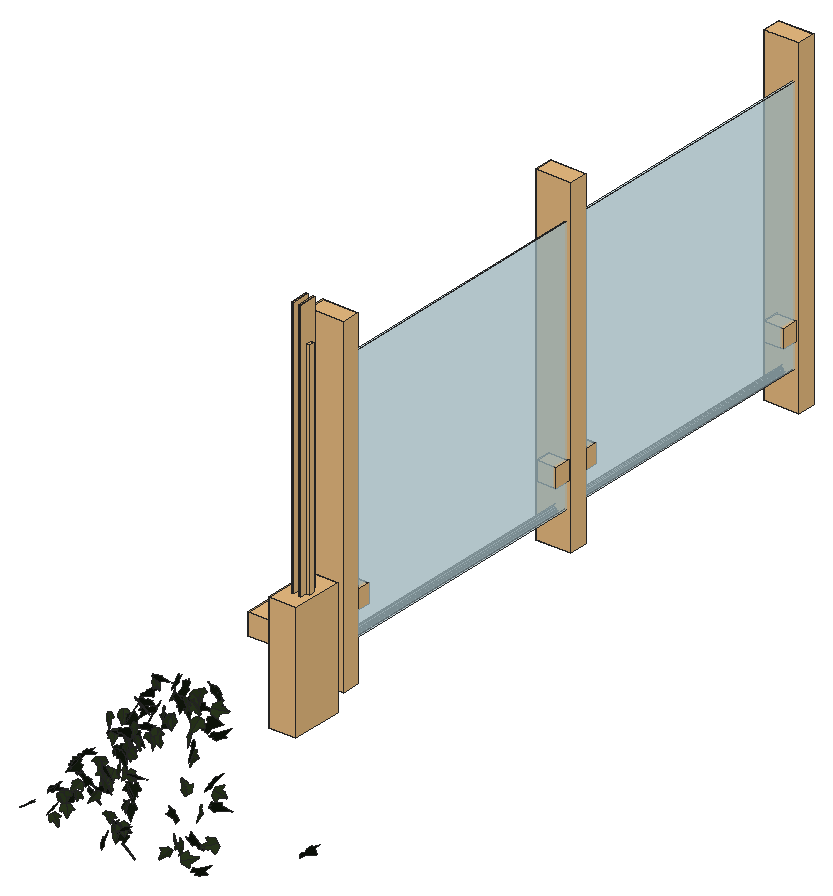
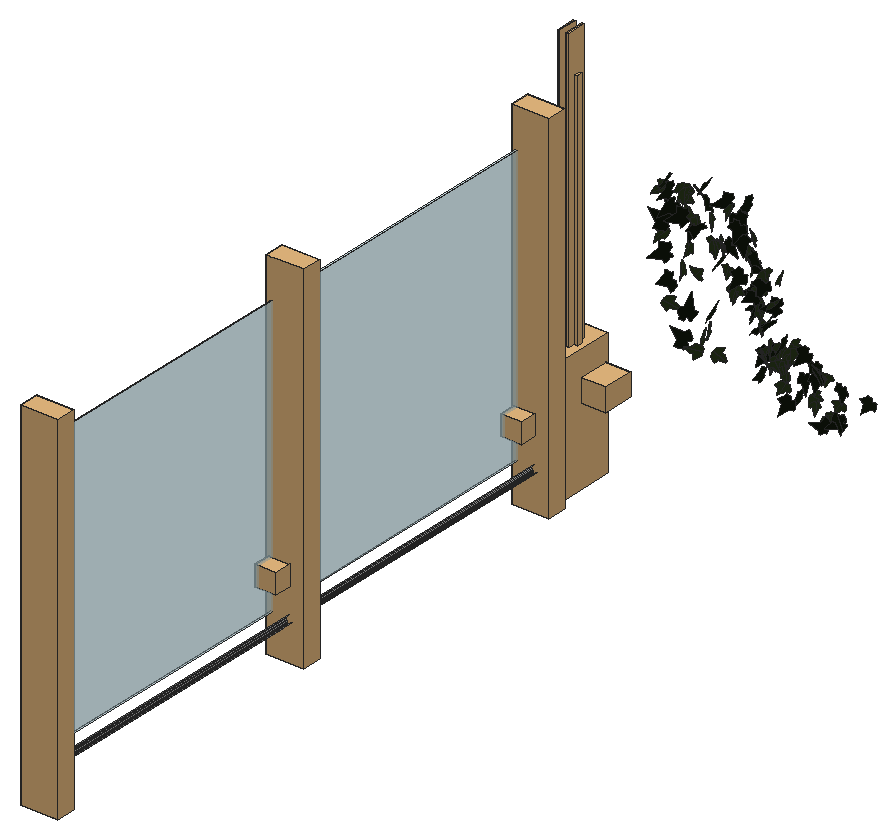
# SketchUp Ruby script. Lengths in inches.
U = 1.inch
M = Sketchup.active_model
def pt(a) = Geom::Point3d.new(a.map { |v| v * U })
def face(e, loops, mat)
  f = e.add_face(loops[0].map { |a| pt(a) })
  loops[1..].each { |l| e.add_face(l.map { |a| pt(a) }).erase! }
  f.material = f.back_material = mat if mat
  f
end
# faces: each face lists its corners as indices into pts; further lists are holes
def faces(e, pts, list, mat = nil) = list.each { |f| face(e, (f[0].is_a?(Array) ? f : [f]).map { |l| l.map { |i| pts[i] } }, mat) }
# xy, xz, yz: faces in a plane at the given z, y or x. An outline is a flat list of corners, or four numbers for a rectangle; further outlines are holes
def ring(l) = l.size == 4 ? [[l[0], l[1]], [l[2], l[1]], [l[2], l[3]], [l[0], l[3]]] : l.each_slice(2).to_a
def flat(e, list, mat, &to3) = list.each { |f| face(e, (f[0].is_a?(Array) ? f : [f]).map { |l| ring(l).map { |u, v| to3.(u, v) } }, mat) }
def xy(e, z, list, mat = nil) = flat(e, list, mat) { |x, y| [x, y, z] }
def xz(e, y, list, mat = nil) = flat(e, list, mat) { |x, z| [x, y, z] }
def yz(e, x, list, mat = nil) = flat(e, list, mat) { |y, z| [x, y, z] }
def lines(e, pts, list) = list.each { |a, b| e.add_line(pt(pts[a]), pt(pts[b])) }
# prism: a flat outline (further loops are holes) pulled along v
def prism(e, loops, v, mat = nil)
  f = face(e, loops, mat); d = Geom::Vector3d.new(v.map { |x| x * U })
  f.pushpull(f.normal.samedirection?(d) ? d.length : -d.length)
end
def box(e, o, s, mat = nil) = prism(e, [[o, [o[0] + s[0], o[1], o[2]], [o[0] + s[0], o[1] + s[1], o[2]], [o[0], o[1] + s[1], o[2]]]], [0, 0, s[2]], mat)
def at(x, y, z, deg = 0) = Geom::Transformation.translation(pt([x, y, z])) * Geom::Transformation.rotation(ORIGIN, Z_AXIS, deg.degrees)
def axes(o, x, y, z) = Geom::Transformation.new([*x, 0, *y, 0, *z, 0, *pt(o).to_a, 1])
def part(name) = M.definitions.add(name)
# library, detail: a bought-in or finely detailed component or shape, given as its bounding box
def library(name, o, s) = part(name).tap { |d| box(d.entities, o, s) }
def detail(e, o, s) = box(e.add_group.entities, o, s)
def put(e, d, t, mat = nil) = e.add_instance(d, t).tap { |i| i.material = mat if mat }
def group(e, t, mat = nil) = e.add_group.tap { |g| g.transformation = t; g.material = mat if mat }.entities
root = M.entities
M.materials.add("Glass Rail Metal").color = [192, 192, 192]
M.materials.add("[Translucent Glass Safety]").color = [204, 235, 244]
M.materials["[Translucent Glass Safety]"].alpha = 0.5
M.materials.add("[Translucent Glass Tinted]").color = [8, 201, 241]
M.materials["[Translucent Glass Tinted]"].alpha = 0.48
M.materials.add("efeu1").color = [18, 25, 13]
M.materials.add("efeu2").color = [43, 57, 29]
c1 = part("ivyleaf_9")
p = [[1.54,2.16,1.25],[1.36,2.04,1.19],[-0.21,0.99,0.68],[-0.71,1.11,0.82],[-0.85,0.86,0.67],[-0.8,0.17,0.21],
  [-0.9,-0.01,0.1],[-0.67,-0.16,-0.02],[-0.08,-0.08,-0.05],[-0.03,-0.6,-0.4],[0.65,-0.88,-0.66],[0.83,-0.6,-0.49],
  [1.29,-0.42,-0.43],[1.8125,-0.07,-0.26],[1.21,0.44,0.15]]
faces(c1.entities,p,[[0,1,2,3,4,5,6,7,8,9,10,11,12,13,14]],"efeu1")
c2 = part("ivyleaf_10")
p = [[0,0.5,-0.03],[-0.0625,2.02,-0.43],[-0.19,2.01,-0.46],[-0.54,1.05,-0.29],[-0.52,0.625,-0.18],[-0.83,0.76,-0.28],
  [-1.16,0.64,-0.33],[-1.15,0.33,-0.24],[-0.77,-0.39,0.02],[-0.3,-0.51,0.16],[0.04,-0.48,0.23],[-0.02,2.01,-0.4375],
  [-0.06,2.01,-0.43],[0.04,-0.49,0.23],[0.67,-0.49,0.14],[1.38,0.36,-0.2],[1.375,0.51,-0.24],[0.81,0.65,-0.19],
  [0.62,0.59,-0.15],[0.6,1.09,-0.28],[0.5,1.23,-0.31]]
faces(c2.entities,p,[[0,1,2,3,4,5,6,7,8,9,10],[11,12,0,13,14,15,16,17,18,19,20]],"efeu2")
c3 = library("glass bracket3\#1",[-0.84,-0.98,-1],[3.67,3.29,2])
c4 = library("Group\#46",[0,0,0],[50.8,6,878.92])
c5 = library("Group\#15",[0.69,0,0.79],[0.62,1.89,30.3])
c6 = library("Group\#43",[0,0,0],[50.8,6,878.92])
c7 = library("Group\#53",[0,0,0],[3.15,5.91,11.14])
c8 = library("Post-Glass-Railing",[-1.57,-2.95,0],[3.14,5.9,36])
c9 = library("Group\#37",[0,0,0],[3.67,3.3,2.01])
c10 = part("Group566\#1")
prism(c10.entities,[[[-0.11,0,0.36],[-0.2,0,0.32],[-0.28,0,0.25],[-0.33,0,0.17],[-0.37,0,0.08],[-0.375,0,-0.02],[-0.36,0,-0.11],[-0.32,0,-0.2],[-0.25,0,-0.28],[-0.17,0,-0.33],[-0.08,0,-0.37],[0.02,0,-0.375],[0.11,0,-0.36],[0.2,0,-0.32],[0.28,0,-0.25],[0.33,0,-0.17],[0.37,0,-0.08],[0.375,0,0.02],[0.36,0,0.11],[0.32,0,0.2],[0.25,0,0.28],[0.17,0,0.33],[0.08,0,0.37],[-0.02,0,0.375]]],[0,46.9,0],"Glass Rail Metal")
c11 = part("Group569\#1")
prism(c11.entities,[[[-0.11,0,0.36],[-0.2,0,0.32],[-0.28,0,0.25],[-0.33,0,0.17],[-0.37,0,0.08],[-0.375,0,-0.02],[-0.36,0,-0.11],[-0.32,0,-0.2],[-0.25,0,-0.28],[-0.17,0,-0.33],[-0.08,0,-0.37],[0.02,0,-0.375],[0.11,0,-0.36],[0.2,0,-0.32],[0.28,0,-0.25],[0.33,0,-0.17],[0.37,0,-0.08],[0.375,0,0.02],[0.36,0,0.11],[0.32,0,0.2],[0.25,0,0.28],[0.17,0,0.33],[0.08,0,0.37],[-0.02,0,0.375]]],[0,46.9,0],"Glass Rail Metal")
box(root,[596.41,193.53,255.11],[0.4,60.48,55.82],"[Translucent Glass Safety]")
box(root,[596.41,254.97,255.11],[0.4,60.48,55.82],"[Translucent Glass Safety]")
put(root,c1,axes([593.52,131.16,242.3],[0.05109,-0.0036,0.99695],[0.23191,0.97092,-0.00838],[-0.96961,0.23203,0.05053]))
put(root,c2,axes([594.59,131.82,248.57],[-0.99335,-0.22111,0.05207],[-0.04736,-0.02687,-1.01754],[0.22217,-0.99435,0.01591]))
put(root,c2,axes([614.49,131.25,255.9],[0.15516,-0.72314,-1.01067],[-0.18535,0.99366,-0.73943],[1.22883,0.24119,0.01609]))
put(root,c2,axes([585.2,131.85,246.64],[0.9105,0.40859,0.19804],[0.14939,0.14949,-0.99524],[-0.42877,0.91972,0.07378]))
put(root,c1,axes([576.93,131.11,244.46],[0.55118,0.72166,0.43785],[-0.02792,0.53823,-0.85196],[-0.84364,0.45367,0.31426]))
put(root,c1,axes([595.92,131.78,247.19],[1.01574,-0.1475,-0.04468],[-0.04343,0.01185,-1.02638],[0.14787,1.01666,0.00548]))
put(root,c2,axes([599.88,132.17,267.16],[0.88384,-0.63502,-0.04472],[-0.03175,0.03245,-1.08828],[0.6358,0.88437,0.00782]))
put(root,c2,axes([598.07,132.23,251.59],[0.31267,-0.96955,0.03657],[0.09794,-0.00669,-1.01464],[0.96529,0.31473,0.0911]))
put(root,c2,axes([597.06,131.84,247.11],[0.50893,0.83618,0.3194],[0.14025,0.28839,-0.97846],[-0.88405,0.52712,0.02865]))
put(root,c2,axes([598.5,131.875,257.6875],[-0.59403,-0.62527,-0.60153],[0.54114,0.30284,-0.8492],[0.67821,-0.7893,0.1507]))
put(root,c1,axes([597.85,132.25,245.51],[-0.9164,0.34409,0.24843],[-0.24197,0.06208,-0.97852],[-0.34867,-0.94745,0.02611]))
put(root,c2,axes([596.23,131.44,244.52],[-0.01474,0.45905,-0.93566],[0.01865,0.93572,0.45878],[1.04203,-0.01025,-0.02145]))
put(root,c1,axes([582.3,131.63,245.32],[-0.09159,0.95753,0.30224],[-0.03807,0.29996,-0.96186],[-1.00337,-0.09879,0.0089]))
put(root,c2,axes([617.91,131.5,261.08],[0.22731,0.68832,0.95487],[0.17961,0.94084,-0.72096],[-1.16331,0.27975,0.07527]))
put(root,c1,axes([600.31,132.16,272.49],[1.00525,-0.47433,-0.01451],[-0.00236,0.029,-1.11125],[0.47455,1.00493,0.02522]))
put(root,c1,axes([597.37,131.57,246.52],[0.60606,0.77669,0.281],[0.13319,0.25207,-0.98399],[-0.81515,0.61865,0.04815]))
put(root,c1,axes([597.45,132.4,242.96],[0.7878,-0.55811,0.16896],[0.14545,-0.08695,-0.96537],[0.56469,0.80101,0.01293]))
put(root,c1,axes([617.02,131.82,257.8],[0.96572,0.2001,0.67518],[0.65709,0.15607,-0.9861],[-0.25325,1.16796,0.01609]))
put(root,c1,axes([612.31,132.86,248.31],[1.18041,-0.40295,0.4183],[-0.37878,0.18419,1.24632],[-0.44031,-1.23871,0.04925]))
put(root,c2,axes([599.14,131.79,261.92],[-0.03977,0.76946,0.74074],[-0.19617,0.72339,-0.76196],[-1.0499,-0.16431,0.11431]))
put(root,c2,axes([591.01,132.94,250.66],[0.03574,0.74348,-0.73897],[-0.5623,-0.61042,-0.64135],[-0.88468,0.41802,0.37778]))
put(root,c1,axes([598.79,132.14,257.2],[0.86505,-0.13114,0.57115],[0.58571,0.22626,-0.83515],[-0.01886,1.0116,0.26084]))
put(root,c1,axes([598.13,132.9375,251.16],[-0.04178,-1.01173,-0.09202],[0.02043,0.09125,-1.01245],[1.0157,-0.04345,0.01658]))
put(root,c1,axes([612.93,132.31,243.45],[0.80863,0.78591,-0.32463],[0.21755,0.24186,1.12743],[0.82202,-0.83712,0.02097]))
put(root,c1,axes([598.71,133,254.95],[-0.31415,-0.93948,-0.29267],[0.15808,0.25505,-0.9884],[0.97123,-0.34539,0.06621]))
put(root,c2,axes([599.52,132.85,264.41],[-0.91904,0.327,-0.44558],[0.37546,-0.26508,-0.96895],[-0.40559,-0.98636,0.11267]))
put(root,c1,axes([598.37,132.43,254.73],[0.751,-0.21212,-0.67541],[-0.5734,0.39521,-0.7617],[0.41519,0.9295,0.16973]))
put(root,c2,axes([616.15,133.16,249.74],[0.53999,0.08734,-1.12827],[-1.11623,-0.1645,-0.54697],[-0.18613,1.23997,0.00691]))
put(root,c2,axes([595.12,132.3,246.05],[0.07212,0.56648,0.83577],[-0.4327,0.77439,-0.48754],[-0.91224,-0.32253,0.29733]))
put(root,c2,axes([581.63,132.86,243.17],[0.83727,0.21181,0.50987],[0.43339,0.32167,-0.84531],[-0.34205,0.92602,0.17702]))
put(root,c2,axes([607.58,133.5,246.68],[-0.66381,0.60662,0.68828],[0.48972,-0.48411,0.89898],[0.77581,0.82463,0.02145]))
put(root,c2,axes([605.66,133.9,244.38],[-0.34268,-0.66613,0.76763],[-0.35991,-0.67806,-0.74907],[0.9505,-0.4969,-0.00689]))
put(root,c2,axes([608.34,134.04,245.97],[-0.3466,0.41747,1.04975],[0.63507,-0.83612,0.5422],[0.93431,0.72319,0.02088]))
put(root,c1,axes([636.56,132.56,255.68],[0.52105,1.17741,0.39801],[0.15925,0.36477,-1.28755],[-1.23262,0.54483,0.0019]))
put(root,c1,axes([601.49,133.85,270.58],[-0.00972,0.81704,-0.74601],[-0.26458,-0.72611,-0.7918],[-1.07429,0.17143,0.20176]))
put(root,c1,axes([607.48,134.82,273.82],[0.05775,-0.96738,0.6452],[0.20014,-0.62809,-0.95963],[1.14545,0.15852,0.13515]))
put(root,c1,axes([606.16,134.85,251.21],[0.61893,-0.76581,-0.4584],[0.28415,-0.35973,0.98464],[-0.84608,-0.68102,-0.00464]))
put(root,c2,axes([609.62,133.99,257.22],[0.91306,0.11017,0.74852],[-0.7524,0.00895,0.91647],[0.0795,-1.18063,0.0768]))
put(root,c2,axes([611.41,134.77,271.09],[0.65116,0.75238,-0.71914],[-0.46123,-0.55184,-0.99498],[-0.933,0.7979,-0.01003]))
put(root,c2,axes([608.98,134.08,243.77],[0.20729,0.0311,-1.17214],[1.12329,0.33613,0.20757],[0.3363,-1.14188,0.02918]))
put(root,c1,axes([609.7,135.57,265.65],[-0.19776,0.04524,-1.1502],[0.9768,-0.61085,-0.19198],[-0.609,-0.99446,0.06559]))
put(root,c2,axes([603.28,134.28,264.3],[0.01283,0.73382,-0.82121],[-0.20926,0.80793,0.71868],[1.08124,0.14765,0.14884]))
put(root,c2,axes([609.01,135.63,267.31],[0.81395,-0.75015,0.35053],[0.25309,-0.24262,-1.10688],[0.78838,0.85237,-0.00657]))
put(root,c2,axes([591,136.16,264.41],[-0.23559,1.00027,-0.31076],[0.04001,-0.30969,-1.02718],[-1.04667,-0.23699,0.03068]))
put(root,c2,axes([609.72,135.5,263.15],[0.00068,-0.68058,-0.94651],[0.02923,0.94622,-0.68035],[1.16542,-0.02333,0.01762]))
put(root,c1,axes([589.72,136.59,253.41],[0.84888,-0.4369,-0.43493],[-0.35681,0.25539,-0.95294],[0.50273,0.91899,0.05806]))
put(root,c1,axes([595.05,137.29,265.24],[-0.51951,-0.36875,-0.89917],[0.87935,0.25577,-0.61295],[0.4138,-1.00647,0.17367]))
put(root,c1,axes([607,137.17,275],[-1.04466,0.52194,0.01236],[-0.01285,0.00195,-1.16778],[-0.52193,-1.04473,0.004]))
put(root,c1,axes([595.73,137.4,266.98],[-0.68714,0.56503,-0.61847],[0.38093,-0.50168,-0.88156],[-0.7461,-0.77652,0.11951]))
put(root,c1,axes([593.9,136.68,262.49],[0.81841,0.68968,-0.24282],[-0.19958,-0.1399,-1.07006],[-0.70341,0.84213,0.0211]))
put(root,c1,axes([600.48,136.93,274.72],[0.9296,-0.04931,0.62228],[0.62357,0.12456,-0.92166],[-0.02864,1.1117,0.13087]))
put(root,c1,axes([597.9375,137.22,269.36],[0.54671,0.65027,-0.69072],[-0.51199,-0.46888,-0.84667],[-0.79863,0.74574,0.06995]))
put(root,c1,axes([612.12,136.54,270.27],[0.06833,0.11823,-1.22233],[-0.32032,1.18356,0.09657],[1.18552,0.31297,0.09654]))
put(root,c2,axes([592.88,137.63,265.1],[0.3397,1.01263,-0.20331],[-0.09215,-0.18345,-1.06771],[-1.02872,0.35082,0.02851]))
put(root,c2,axes([600.1875,137.16,273.97],[-0.16121,1.04009,0.36399],[-0.04802,0.36088,-1.05249],[-1.1009,-0.16804,-0.00739]))
put(root,c1,axes([598.45,137.02,271.16],[0.47335,0.98786,0.11357],[0.03676,0.10831,-1.09532],[-0.99368,0.47458,0.01358]))
put(root,c2,axes([579.29,137.79,243.91],[-0.80452,0.15219,-0.61559],[0.56277,-0.28695,-0.80643],[-0.29224,-0.97153,0.14175]))
put(root,c1,axes([583.15,138,251.57],[-1.02198,0.12001,0.16733],[-0.16614,0.01988,-1.02901],[-0.12165,-1.0354,-0.00036]))
put(root,c1,axes([591.86,138.08,256.67],[0.52935,-0.95965,0.0234],[0.0235,-0.01376,-1.09588],[0.95965,0.52969,0.01393]))
put(root,c2,axes([590.74,137.86,260.3125],[0.36461,0.97253,-0.19472],[-0.12438,-0.16099,-1.03696],[-0.984,0.38071,0.05892]))
put(root,c2,axes([609.15,137.79,274.75],[-0.82422,-0.81256,-0.11223],[0.10246,0.05587,-1.15696],[0.81385,-0.82994,0.03199]))
put(root,c2,axes([613.26,137.05,273.07],[0.15591,0.38876,1.18079],[0.5091,1.0657,-0.41809],[-1.13412,0.53183,-0.02536]))
put(root,c2,axes([608.67,138.05,274.17],[-0.34022,-1.1092,0.03978],[0.36119,-0.14998,-1.09302],[1.0495,-0.30795,0.38906]))
put(root,c2,axes([602.87,137.99,267.32],[1.10219,-0.07402,0.25396],[0.26179,0.14926,-1.0927],[0.03792,1.12118,0.16224]))
put(root,c1,axes([599.7,138.25,268.36],[-0.63461,0.6911,-0.64158],[0.42375,-0.48186,-0.9382],[-0.84243,-0.763,0.01139]))
put(root,c1,axes([582.68,137.89,252.1],[-0.3812,0.91992,-0.26859],[0.08289,-0.25632,-0.99556],[-0.95474,-0.38955,0.02081]))
put(root,c1,axes([612.67,137.66,267.25],[0.74395,0.94941,-0.34969],[0.20687,0.28214,1.20612],[0.99039,-0.7721,0.01074]))
put(root,c2,axes([601.26,138.12,268.15],[0.63196,-0.88658,-0.11473],[0.03597,0.1656,-1.0816],[0.89325,0.62057,0.12472]))
put(root,c2,axes([599.7,138.15,263.57],[1.04415,-0.0017,0.4011],[0.3961,0.18066,-1.03034],[-0.06322,1.10386,0.16924]))
put(root,c1,axes([584.64,137.98,249.38],[0.65827,0.26493,-0.7795],[-0.73478,-0.26112,-0.70925],[-0.37135,0.98628,0.02161]))
put(root,c1,axes([590.11,137.78,259.86],[0.82539,0.01301,0.69398],[0.66579,0.28996,-0.79731],[-0.19621,1.03866,0.21388]))
put(root,c2,axes([582.31,138.79,247.15],[0.36101,0.55538,-0.76273],[-0.49291,-0.58534,-0.65952],[-0.80452,0.60784,0.06181]))
put(root,c2,axes([602.46,138.44,267.13],[-0.09303,-1.12959,-0.04249],[0.02732,0.04038,-1.13316],[1.13005,-0.09397,0.02389]))
put(root,c2,axes([592.72,138.59,259.87],[-0.79236,0.42248,-0.63949],[0.50578,-0.40287,-0.89284],[-0.57587,-0.93514,0.09573]))
put(root,c2,axes([593.34,138.65,258.9],[-0.00945,-1.05869,0.08056],[0.03084,-0.0808,-1.05826],[1.0613,-0.00708,0.03147]))
put(root,c2,axes([582.34,138.3125,245.61],[-0.99781,0.13306,0.2763],[-0.27162,0.05316,-1.00651],[-0.14237,-1.03399,-0.01619]))
put(root,c1,axes([582.11,138.05,251.24],[-0.35116,0.80842,0.52756],[-0.26242,0.4603,-0.88003],[-0.92898,-0.43562,0.04917]))
put(root,c1,axes([582,138.23,250.45],[0.72827,0.40307,-0.59217],[-0.59293,-0.13467,-0.82086],[-0.40196,0.92893,0.13795]))
put(root,c2,axes([607.07,138.64,271.23],[0.65171,-0.07385,0.94765],[0.94756,0.14119,-0.64064],[-0.07505,1.14142,0.14056]))
put(root,c1,axes([593.43,138.34,259.63],[0.93673,-0.1931,-0.46559],[-0.4362,0.18181,-0.953],[0.25258,1.03014,0.08091]))
put(root,c1,axes([591.17,138.84,257.0625],[0.19836,-0.94925,-0.41107],[0.08133,0.43158,-0.95735],[1.03123,0.14856,0.15457]))
put(root,c1,axes([611.57,139.13,275.48],[0.60554,-0.99144,0.14789],[0.09713,-0.11393,-1.1615],[0.99769,0.61284,0.02332]))
put(root,c1,axes([611.49,137.78,257.43],[-0.36595,0.85929,-0.84948],[-0.32794,0.78364,0.93396],[1.16295,0.49138,-0.00394]))
put(root,c1,axes([594.15,138.77,260.93],[-0.08248,-0.22134,-1.041],[0.84221,0.62477,-0.19957],[0.65067,-0.83675,0.12636]))
put(root,c2,axes([590.99,138.86,253.4375],[0.47807,-0.96265,-0.08008],[0.16643,0.1701,-1.0512],[0.95153,0.4539,0.22409]))
put(root,c2,axes([602.92,138.67,271.99],[0.31453,-0.97288,-0.4263],[-0.11644,0.41034,-1.02236],[1.05578,0.33509,0.01424]))
put(root,c2,axes([587.68,138.87,251.57],[-0.46549,-0.91247,-0.12137],[0.22756,0.01771,-1.00594],[0.89193,-0.48073,0.19331]))
put(root,c2,axes([579.34,138.89,244.13],[-0.81755,-0.56385,-0.01805],[0.0679,-0.0668,-0.98872],[0.56004,-0.81501,0.09352]))
put(root,c2,axes([586.9,138.875,253.4],[-0.71631,-0.74428,0.00579],[-0.00321,-0.00494,-1.03298],[0.7443,-0.71631,0.00111]))
put(root,c1,axes([577.43,138.4375,244.89],[-0.08228,0.99517,0.0254],[-0.03336,0.02271,-0.99807],[-0.99493,-0.08306,0.03136]))
put(root,c1,axes([603.8,138.05,273.95],[0.11798,0.63617,0.90572],[-0.19188,0.90882,-0.61334],[-1.09006,-0.09112,0.20599]))
put(root,c2,axes([587.17,138.81,252.67],[0.03908,1.03091,0.06279],[-0.00246,0.06293,-1.03164],[-1.03282,0.03886,0.00483]))
put(root,c1,axes([584.07,138.19,253.875],[0.61235,0.69984,0.47488],[0.24406,0.41513,-0.92648],[-0.80977,0.65433,0.07987]))
put(root,c2,axes([605.8,138.89,270.77],[-0.98577,0.38988,0.45301],[-0.50208,-0.06614,-1.03562],[-0.32425,-1.08286,0.22635]))
put(root,c1,axes([596.87,138.45,263.58],[0.92972,0.54423,0.06894],[0.03756,0.07219,-1.07643],[-0.5473,0.92948,0.04324]))
put(root,c1,axes([584.71,138.94,246.41],[0.88239,-0.51416,-0.24126],[-0.1498,0.21927,-1.01521],[0.54783,0.88811,0.11099]))
put(root,c2,axes([587.29,139.05,252.05],[-0.77424,0.67422,0.12444],[-0.19679,-0.03873,-1.01453],[-0.65676,-0.78322,0.15729]))
put(root,c1,axes([576.68,138.57,244.22],[0.71001,0.32048,0.63042],[0.50692,0.39226,-0.77033],[-0.49312,0.86468,0.1158]))
put(root,c2,axes([587.58,139.08,249.22],[-0.94634,0.43212,0.20093],[-0.19846,0.04881,-1.03966],[-0.43326,-0.96621,0.03734]))
put(root,c1,axes([600.32,140.31,264.87],[-0.26038,-0.71974,0.82282],[0.09602,-0.85762,-0.7198],[1.08896,-0.09647,0.26021]))
put(root,c2,axes([597.45,139.36,261.39],[-1.04902,-0.30508,-0.21695],[0.23046,-0.01764,-1.08956],[0.295,-1.07107,0.07974]))
put(root,c2,axes([597.09,139.66,260.65],[-0.71291,0.81841,-0.22686],[0.14382,-0.17558,-1.08535],[-0.83701,-0.72724,0.00674]))
put(root,c2,axes([588.84,139.81,251.15],[0.94721,0.36869,-0.33995],[-0.34969,-0.03519,-1.01251],[-0.35946,1.00575,0.08919]))
put(root,c1,axes([607.51,139.48,270.67],[0.93316,0.05882,0.67245],[0.67045,0.05245,-0.93497],[-0.07837,1.14901,0.00825]))
put(root,c2,axes([591.53,139.98,252.12],[0.77499,-0.71395,-0.2171],[-0.17865,0.12638,-1.05337],[0.72453,0.79484,-0.02752]))
put(root,c1,axes([579.2,139.5,242.81],[0.12831,0.07802,0.98269],[0.94072,0.28649,-0.14558],[-0.29463,0.94872,-0.03686]))
put(root,c1,axes([604.59,140.26,270.375],[-0.24615,-1.0055,-0.48905],[0.11648,0.47498,-1.03519],[1.11204,-0.27232,0.00017]))
put(root,c1,axes([609.75,140.2,275.125],[1.06059,-0.47378,0.069],[0.05978,-0.03535,-1.16157],[0.47503,1.06224,-0.00788]))
put(root,c2,axes([586.68,140.64,248.36],[-0.8389,-0.40827,-0.49554],[0.53215,0.01408,-0.91248],[0.35925,-0.97423,0.19448]))
put(root,c1,axes([585.14,141.15,246.2],[0.85744,0.58964,0.10067],[0.05376,0.09927,-1.03936],[-0.59575,0.8576,0.0511]))
put(root,c3,axes([590.29,178.46,263.56],[1.9,0,0],[0,1.9,0],[0,0,2.261]),"[Translucent Glass Tinted]")
put(root,c4,axes([597.75,179.56,248.78],[0,0.0748,0],[-0.0748,0,0.00001],[0.00001,0,0.08902]),"[Translucent Glass Tinted]")
put(root,c5,axes([598.5,179.56,248.78],[0,1.9,0],[-1.9,0,0.00031],[0.00026,0,2.261]),"Glass Rail Metal")
put(root,c6,axes([596.11,179.56,248.78],[0,0.0748,0],[-0.0748,0,0.00001],[0.00001,0,0.08902]),"[Translucent Glass Tinted]")
put(root,c7,axes([593.71,175.85,245.62],[1.9,0,0],[0,1.9,0],[0,0,2.261]),"[Translucent Glass Tinted]")
put(root,c8,axes([593.9375,193.05,247.11],[0,1.28,0],[-1.28,0,0],[0,0,1.99144]))
put(root,c9,axes([597.22,193.77,260.92],[0,1.28,0],[-1.28,0,0],[0,0,1.99144]),"[Translucent Glass Safety]")
put(root,c10,axes([593.9375,193.75,254.17],[1.28,0,0],[0,1.28,0],[0,0,1.99144]))
put(root,c9,axes([597.22,253.79,264.91],[0,-1.28,0.00027],[-1.28,0,0],[0,-0.00017,-1.99144]),"[Translucent Glass Safety]")
put(root,c8,axes([593.9375,254.49,247.11],[0,1.28,0],[-1.28,0,0],[0,0,1.99144]))
put(root,c9,axes([597.22,255.21,260.92],[0,1.28,0],[-1.28,0,0],[0,0,1.99144]),"[Translucent Glass Safety]")
put(root,c11,axes([593.9375,255.19,254.17],[1.28,0,0],[0,1.28,0],[0,0,1.99144]))
put(root,c9,axes([597.22,315.23,264.91],[0,-1.28,0.00027],[-1.28,0,0],[0,-0.00017,-1.99144]),"[Translucent Glass Safety]")
put(root,c8,axes([593.9375,315.93,247.11],[0,1.28,0],[-1.28,0,0],[0,0,1.99144]))
